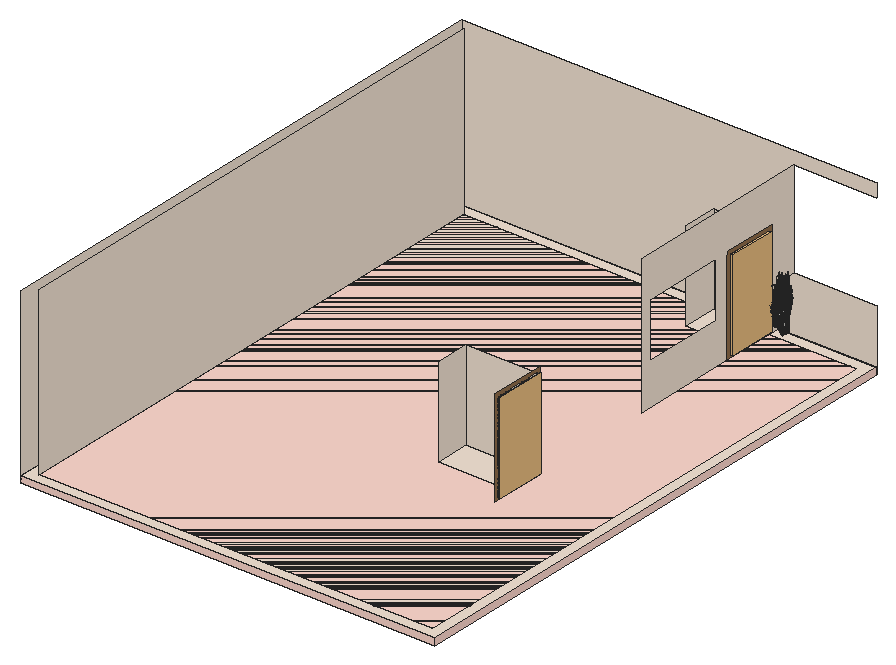
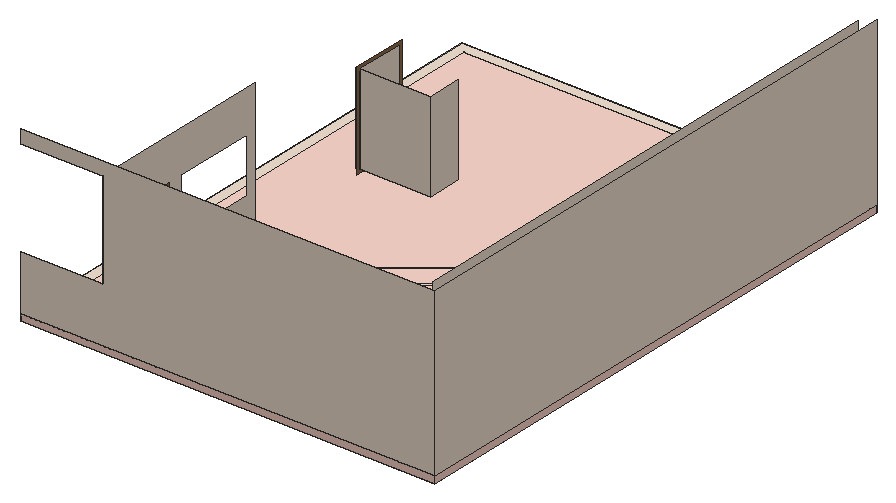
# SketchUp Ruby script. Lengths in inches.
U = 1.inch
M = Sketchup.active_model
def pt(a) = Geom::Point3d.new(a.map { |v| v * U })
def face(e, loops, mat)
  f = e.add_face(loops[0].map { |a| pt(a) })
  loops[1..].each { |l| e.add_face(l.map { |a| pt(a) }).erase! }
  f.material = f.back_material = mat if mat
  f
end
# faces: each face lists its corners as indices into pts; further lists are holes
def faces(e, pts, list, mat = nil) = list.each { |f| face(e, (f[0].is_a?(Array) ? f : [f]).map { |l| l.map { |i| pts[i] } }, mat) }
# xy, xz, yz: faces in a plane at the given z, y or x. An outline is a flat list of corners, or four numbers for a rectangle; further outlines are holes
def ring(l) = l.size == 4 ? [[l[0], l[1]], [l[2], l[1]], [l[2], l[3]], [l[0], l[3]]] : l.each_slice(2).to_a
def flat(e, list, mat, &to3) = list.each { |f| face(e, (f[0].is_a?(Array) ? f : [f]).map { |l| ring(l).map { |u, v| to3.(u, v) } }, mat) }
def xy(e, z, list, mat = nil) = flat(e, list, mat) { |x, y| [x, y, z] }
def xz(e, y, list, mat = nil) = flat(e, list, mat) { |x, z| [x, y, z] }
def yz(e, x, list, mat = nil) = flat(e, list, mat) { |y, z| [x, y, z] }
def lines(e, pts, list) = list.each { |a, b| e.add_line(pt(pts[a]), pt(pts[b])) }
# prism: a flat outline (further loops are holes) pulled along v
def prism(e, loops, v, mat = nil)
  f = face(e, loops, mat); d = Geom::Vector3d.new(v.map { |x| x * U })
  f.pushpull(f.normal.samedirection?(d) ? d.length : -d.length)
end
def box(e, o, s, mat = nil) = prism(e, [[o, [o[0] + s[0], o[1], o[2]], [o[0] + s[0], o[1] + s[1], o[2]], [o[0], o[1] + s[1], o[2]]]], [0, 0, s[2]], mat)
def at(x, y, z, deg = 0) = Geom::Transformation.translation(pt([x, y, z])) * Geom::Transformation.rotation(ORIGIN, Z_AXIS, deg.degrees)
def axes(o, x, y, z) = Geom::Transformation.new([*x, 0, *y, 0, *z, 0, *pt(o).to_a, 1])
def part(name) = M.definitions.add(name)
# library, detail: a bought-in or finely detailed component or shape, given as its bounding box
def library(name, o, s) = part(name).tap { |d| box(d.entities, o, s) }
def detail(e, o, s) = box(e.add_group.entities, o, s)
def put(e, d, t, mat = nil) = e.add_instance(d, t).tap { |i| i.material = mat if mat }
def group(e, t, mat = nil) = e.add_group.tap { |g| g.transformation = t; g.material = mat if mat }.entities
root = M.entities
M.materials.add("B01_Ivory_Dust").color = [255, 217, 206]
M.materials.add("C01_Vanilla_Cream").color = [244, 228, 212]
M.materials.add("LightPink_Translucent").color = [144, 107, 117]
M.materials["LightPink_Translucent"].alpha = 0.75
M.materials.add("Wood_Floor_01_1K").color = [146, 111, 76]
c1 = part("Group\#10")
box(c1.entities,[0,0,0],[360,480,6])
c2 = library("porta+4",[0.2,-5.42,1.33],[46.55,4.72,83.21])
c3 = part("blade")
p = [[2.15,0.21,22],[0,0.17,0],[0.09,0.45,0],[2.18,0.31,22],[2.29,0.31,22],[0.38,0.45,0],
  [2.48,0.24,33],[2.49,0.24,33],[2.48,0.22,33]]
faces(c3.entities,p,[[0,1,2,3],[4,5,2,3],[6,3,4,7],[8,0,3,6]])
c4 = part("seeds")
p = [[0.3,-0.1,1.38],[-0.01,-0.03,1.59],[-0.01,-0.03,0.03],[0.14,-0.07,-0.07],[0.29,-0.03,3],[0.15,0.01,3.11]]
faces(c4.entities,p,[[0,1,2,3],[1,0,4,5]],"LightPink_Translucent")
c5 = part("blade with seeds")
put(c5.entities,c3,at(0,0,0))
put(c5.entities,c4,axes([2.4,0.25,30.99],[1.5799,-0.05474,1.17369],[-0.12525,1.92788,0.29478],[-0.07173,-0.02425,1.56792]))
xy(root,96,[[288,324,290,396]],"C01_Vanilla_Cream")
xy(root,144,[[[0,0,360,480],[9,9,351,471]]],"C01_Vanilla_Cream")
xy(root,150,[[[0,0,360,480],[9,9,351,471]],[9,9,351,471]],"C01_Vanilla_Cream")
xy(root,165,[[226.53,171,288,201],[240,423,288,453]],"C01_Vanilla_Cream")
xz(root,201,[[226.53,165,288,243]],"C01_Vanilla_Cream")
xz(root,453,[[240,165,288,243]],"C01_Vanilla_Cream")
xz(root,480,[[0,150,0,294,360,294,360,282,288,282,288,198,360,198,360,150]],"C01_Vanilla_Cream")
yz(root,0,[[0,150,480,294]],"C01_Vanilla_Cream")
yz(root,9,[[9,150,471,294]],"C01_Vanilla_Cream")
yz(root,226.53,[[171,165,201,243]],"C01_Vanilla_Cream")
yz(root,240,[[423,165,453,243]],"C01_Vanilla_Cream")
yz(root,288,[[[314.71,162,408,162,408,246,456,246,456,162,468,162,468,198,480,198,480,282,314.71,282],[324,198,396,246]],[159,165,201,243],[411,165,453,243]],"C01_Vanilla_Cream")
yz(root,288,[[[156,162,204,246],[159,165,201,243]],[[408,162,456,246],[411,165,453,243]]],"Wood_Floor_01_1K")
put(root,c1,at(0,0,144),"B01_Ivory_Dust")
put(root,c2,axes([291.16,410.82,163.74],[0,0.8978,0],[0.58403,0,0],[0,0,0.94]),"C01_Vanilla_Cream")
put(root,c5,axes([295.36,458.6,164.91],[0.23093,-0.01116,1.28532],[-0.15319,0.4836,0.10393],[-0.32909,-0.02991,0.54946]))
put(root,c5,axes([295.45,459.45,164.91],[0.19317,-0.10421,1.28532],[0.16263,0.48153,0.10393],[-0.30326,0.10883,0.54946]))
put(root,c5,axes([294.85,460.27,163.94],[0.19348,0.04044,1.07251],[0.1247,0.41309,-0.23066],[-0.26282,0.07733,0.45856]))
put(root,c2,axes([289.83,157.29,163.73],[0,0.9504,0],[-0.24166,0,0],[0,0,0.9416]),"C01_Vanilla_Cream")
put(root,c5,axes([296.5625,458.95,164.51],[0.15825,-0.07127,1.32798],[0.05457,0.4976,0.10393],[-0.34278,0.06603,0.47463]))
put(root,c5,axes([294.86,459.28,165.54],[-0.09091,0.06396,1.31208],[0.00773,0.46734,-0.2075],[-0.20839,0.06078,0.10523]))
put(root,c5,axes([296.05,458.15,165.74],[-0.55654,-0.01186,-0.53284],[0.03738,-0.49951,0.0643],[-0.23578,-0.05271,0.75375]))
put(root,c5,axes([295.6,458.27,163.94],[0.1087,0.13716,1.07251],[-0.25048,0.37284,-0.23066],[-0.25719,-0.08912,0.45856]))
put(root,c5,axes([295.15,459.02,165.39],[-0.46269,-0.13744,-0.2656],[0.13495,-0.40096,0.3429],[-0.18628,0.03677,0.65611]))
put(root,c5,axes([295.79,457.83,164.91],[0.2068,0.08488,1.28532],[-0.42797,0.35609,0.10393],[-0.26673,-0.16064,0.54946]))
put(root,c5,axes([293.85,459.76,165.53],[0.07105,0.01321,1.33037],[0.2198,0.43529,-0.12571],[-0.14545,0.11425,0.23543]))
put(root,c5,axes([295.47,459.22,165.51],[-0.15083,0.44814,-0.38324],[-0.51712,-0.15361,-0.29685],[-0.2082,0.04109,0.7333]))
put(root,c5,axes([295.86,458.25,165.51],[-0.40426,0.32635,-0.38324],[-0.35404,-0.34474,-0.29685],[-0.2054,-0.04965,0.7333]))
put(root,c5,axes([295.21,459.19,163.12],[0.01412,0.07764,1.32257],[-0.28464,0.40547,-0.20205],[-0.20218,-0.02044,0.22528]))
put(root,c5,axes([295.29,457.34,165.53],[0.04127,0.04917,1.33037],[-0.19898,0.44196,-0.12571],[-0.20151,0.0032,0.23543]))
put(root,c5,axes([294.45,461.14,164.07],[0.23202,-0.22328,0.86145],[0.09155,0.35348,0.63294],[-0.16768,0.06329,0.18974]))
put(root,c5,axes([295.75,457.04,165.54],[-0.11979,-0.00348,1.31208],[-0.38137,0.34775,-0.2075],[-0.20349,-0.07106,0.10523]))
put(root,c5,axes([295.26,458.97,165.55],[0.15729,-0.44921,0.36002],[0.51712,0.15361,0.29685],[-0.20336,0.027,0.74497]))
put(root,c5,axes([295.44,458.84,165.78],[0.28012,0.44611,-0.0912],[-0.49717,0.21923,-0.50621],[-0.20951,0.05886,0.76918]))
put(root,c5,axes([296.07,457.91,165.78],[-0.02981,0.50103,-0.0912],[-0.56442,-0.01369,-0.50621],[-0.21738,-0.0348,0.76918]))
put(root,c5,axes([295.71,457.95,165.39],[-0.31678,-0.30846,-0.2656],[0.36171,-0.29199,0.3429],[-0.18378,-0.04443,0.65611]))
put(root,c5,axes([295.22,458.85,165.55],[-0.20448,-0.33592,0.04823],[0.37288,-0.16442,0.37966],[-0.16437,0.03244,0.57892]))
put(root,c5,axes([296.16,459.78,164.91],[0.13906,-0.15138,1.28532],[0.35111,0.40859,0.10393],[-0.24082,0.18608,0.54946]))
put(root,c5,axes([295.32,460.17,165.39],[-0.48462,0.07041,-0.2656],[-0.12797,-0.4025,0.3429],[-0.13888,0.10811,0.65611]))
put(root,c5,axes([295.06,461.37,163.12],[0.07468,0.04922,1.32257],[0.12663,0.45605,-0.20205],[-0.16551,0.09725,0.22528]))
put(root,c5,axes([294.95,458.6875,164.07],[0.35544,-0.03525,0.86145],[-0.22547,0.31061,0.63294],[-0.17565,-0.04659,0.18974]))
put(root,c5,axes([295.38,460.09,165.55],[-0.13808,-0.45342,0.36002],[0.54163,-0.07869,0.29685],[-0.15963,0.10664,0.74497]))
put(root,c5,axes([295.66,457.83,165.82],[0.45978,-0.36358,0.40322],[0.39653,0.38611,0.33247],[-0.21571,-0.06707,0.83437]))
put(root,c5,axes([295.28,460,165.55],[-0.3822,-0.20719,0.04823],[0.22252,-0.29505,0.37966],[-0.12254,0.09539,0.57892]))
put(root,c5,axes([296.05,460.15,164.91],[0.10366,-0.16934,1.28532],[0.43488,0.35044,0.10393],[-0.19618,0.21841,0.54946]))
put(root,c5,axes([295.64,458.97,165.79],[0.46269,0.13744,0.2656],[-0.13495,0.40096,-0.3429],[-0.18628,0.03677,0.65611]))
put(root,c5,axes([295.72,460.22,165.51],[0.14302,0.44985,-0.38324],[-0.54163,0.07869,-0.29685],[-0.15522,0.12083,0.7333]))
put(root,c5,axes([295.875,457.83,165.55],[0.02803,-0.37463,0.04823],[0.42332,0.01027,0.37966],[-0.16216,-0.0392,0.57892]))
put(root,c5,axes([294.875,461.03,165.54],[-0.01384,0.09749,1.31208],[0.39274,0.33916,-0.2075],[-0.10282,0.16039,0.10523]))
put(root,c5,axes([297.07,459.9,163.54],[-0.57914,-0.08077,-0.46765],[0.12221,-0.49823,-0.12274],[-0.17283,-0.06037,1.03225]))
put(root,c5,axes([297.18,457.18,166.07],[-0.37157,0.4723,-0.10215],[-0.5381,-0.2721,-0.56695],[-0.18705,-0.13344,0.86148]))
put(root,c5,axes([296.16,458.11,165.79],[0.31678,0.30846,0.2656],[-0.36171,0.29199,-0.3429],[-0.18378,-0.04443,0.65611]))
put(root,c5,axes([297.01,457.5625,165.74],[-0.47473,-0.23813,-0.53284],[0.33738,-0.41728,0.0643],[-0.172,-0.14218,0.75375]))
put(root,c5,axes([296.79,457.58,165.51],[-0.54938,0.11711,-0.38324],[-0.0961,-0.44351,-0.29685],[-0.14756,-0.1271,0.7333]))
put(root,c5,axes([296.3125,460.84,163.51],[-0.52105,-0.24633,-0.37238],[0.31144,-0.44171,0],[-0.11867,-0.0561,1.18128]))
put(root,c5,axes([296.08,457.17,163.12],[-0.05393,0.0649,1.32257],[-0.545,0.13993,-0.20205],[-0.13166,-0.12729,0.22528]))
put(root,c5,axes([295.47,459.9,165.78],[0.515,0.27165,-0.0912],[-0.2967,0.3934,-0.50621],[-0.1455,0.13675,0.76918]))
put(root,c5,axes([296.63,461.14,163.78],[-0.34808,0.49367,0],[-0.58235,-0.27531,-0.38706],[-0.13264,-0.0627,1.22783]))
put(root,c5,axes([294.62,461.08,166.23],[0.49129,0.13151,-0.04866],[-0.15113,0.40475,-0.22062],[-0.08035,0.06145,0.72768]))
put(root,c5,axes([295.72,459.94,165.79],[0.48462,-0.07041,0.2656],[0.12797,0.4025,-0.3429],[-0.13888,0.10811,0.65611]))
put(root,c5,axes([295.99,461.85,163.94],[0.17569,-0.07772,1.07251],[0.43377,0.23434,-0.23066],[-0.12911,0.20277,0.45856]))
put(root,c5,axes([295.74,457.42,163.6],[-0.1606,0.40228,-0.02919],[-0.4943,-0.12375,-0.13237],[-0.07505,-0.0658,0.43661]))
put(root,c5,axes([297.03,456.06,165.53],[-0.01039,0.05905,1.33037],[-0.51226,0.21431,-0.12571],[-0.15074,-0.10955,0.23543]))
put(root,c5,axes([296.48,456.91,163.94],[-0.03371,0.16116,1.07251],[-0.49286,0.13491,-0.23066],[-0.11521,-0.20831,0.45856]))
put(root,c5,axes([296.64,457.33,164.91],[0.12726,0.15818,1.28532],[-0.58807,0.13317,0.10393],[-0.13291,-0.24832,0.54946]))
put(root,c5,axes([297.73,459.97,164],[-0.56211,0.32708,-0.21822],[-0.3738,-0.46216,-0.37502],[-0.13869,-0.04694,1.19781]))
put(root,c5,axes([296.18,461,165.55],[-0.39645,-0.33614,0.36002],[0.42102,-0.2899,0.29685],[-0.07313,0.15771,0.74497]))
put(root,c5,axes([296.85,457.25,165.39],[-0.08599,-0.39682,-0.2656],[0.49155,-0.10478,0.3429],[-0.13203,-0.11372,0.65611]))
put(root,c5,axes([295.48,459.26,163.78],[-0.69617,0,0],[0,-0.55062,-0.38706],[0,-0.12541,1.22783]))
put(root,c5,axes([296.46,460.66,163.52],[-0.13078,-0.42928,-0.23233],[0.51941,-0.1219,0.23233],[-0.10471,-0.0495,1.0423]))
put(root,c5,axes([296.03,460.97,165.55],[-0.45752,-0.02296,0.04823],[0.01254,-0.34663,0.37966],[-0.04787,0.13278,0.57892]))
put(root,c5,axes([296.17,461.1,165.39],[-0.3767,0.25939,-0.2656],[-0.3566,-0.29618,0.3429],[-0.05426,0.15048,0.65611]))
put(root,c5,axes([298.1,460.33,163.54],[-0.375,0.3703,-0.46765],[-0.46584,-0.33578,-0.12274],[-0.15027,0.09237,1.03225]))
put(root,c5,axes([297.14,457.57,165.79],[0.08599,0.39682,0.2656],[-0.49155,0.10478,-0.3429],[-0.13203,-0.11372,0.65611]))
put(root,c5,axes([294.83,462.03,165.53],[0.06316,-0.02974,1.33037],[0.52204,0.19785,-0.12571],[-0.01227,0.16473,0.23543]))
put(root,c5,axes([296.02,459.11,163.75],[-0.51786,0.4142,0.23067],[-0.51817,-0.40984,-0.27369],[-0.01808,-0.11762,1.23664]))
put(root,c5,axes([298.15,460.26,164.49],[0.48111,0.19866,1.13446],[-0.47133,0.42798,0.44862],[-0.21112,-0.25366,0.95105]))
put(root,c5,axes([296.3125,456.65,164.07],[0.29042,0.17147,0.86145],[-0.42295,0.10307,0.63294],[-0.0905,-0.13178,0.18974]))
put(root,c5,axes([298.36,460.12,163.85],[-0.54364,-0.39653,-0.18894],[0.45745,-0.44527,0.41347],[-0.14639,0.04639,1.26162]))
put(root,c5,axes([297.37,459.74,163.66],[-0.33445,-0.41351,-0.33554],[0.50659,-0.29119,0.16149],[-0.10823,-0.05117,1.07733]))
put(root,c5,axes([296.43,460.83,166],[-0.01449,0.45571,-0.59145],[-0.61002,-0.03061,0.07138],[-0.06438,0.19306,0.83667]))
put(root,c5,axes([296.41,462.11,164.07],[-0.01441,-0.29294,0.86145],[0.36003,0.20894,0.63294],[-0.07081,0.13963,0.18974]))
put(root,c5,axes([296.92,457.1,165.82],[0.62019,-0.12663,0.40322],[0.10763,0.49673,0.33247],[-0.14586,-0.1464,0.83437]))
put(root,c5,axes([298.08,460.04,163.66],[-0.60457,0.03041,-0.33554],[-0.05467,-0.50484,0.16149],[-0.10823,0.05117,1.07733]))
put(root,c5,axes([297.0625,457.21,165.55],[0.25304,-0.31296,0.04823],[0.36033,0.18221,0.37966],[-0.11649,-0.10034,0.57892]))
put(root,c5,axes([296.93,460.88,163.86],[0.52105,0.24633,0.37238],[-0.31144,0.44171,0],[-0.11867,-0.0561,1.18128]))
put(root,c5,axes([296.22,461.47,164.52],[0.01223,-0.25433,1.15759],[0.55017,0.13434,0.15997],[-0.04767,0.27105,0.54661]))
put(root,c5,axes([297.42,459.98,163.83],[0.14756,-0.58378,-0.17572],[0.69966,0.10176,0.38453],[-0.12225,-0.08062,1.1733]))
put(root,c5,axes([297.68,460.11,163.96],[-0.1074,0.43968,0.1086],[-0.52474,-0.07632,-0.3101],[-0.0955,-0.04515,0.95058]))
put(root,c5,axes([297.61,456.28,165.54],[-0.08515,-0.06907,1.31208],[-0.56828,0.04379,-0.2075],[-0.0907,-0.16522,0.10523]))
put(root,c5,axes([298.72,461.34,163.51],[-0.52105,0.24633,-0.37238],[-0.31144,-0.44171,0],[-0.11867,0.0561,1.18128]))
put(root,c5,axes([295.63,458.88,163.51],[0,-0.49266,-0.37238],[0.62289,0,0],[0,-0.11221,1.18128]))
put(root,c5,axes([295.9,459.34,163.86],[0,0.49266,0.37238],[-0.62289,0,0],[0,-0.11221,1.18128]))
put(root,c5,axes([298.75,461.21,163.64],[-0.34375,-0.4954,-0.03857],[0.58235,-0.27531,0.38706],[-0.1435,0.04717,1.22723]))
put(root,c5,axes([296.55,460.98,165.75],[0.39855,0.33102,-0.4254],[-0.42102,0.2899,-0.32951],[-0.06064,0.16819,0.81396]))
put(root,c5,axes([298.6,461.14,163.52],[-0.51941,-0.1219,-0.23233],[0.13078,-0.42928,0.23233],[-0.10471,0.0495,1.0423]))
put(root,c5,axes([296.37,460.74,165.79],[0.3767,-0.25939,0.2656],[0.3566,0.29618,-0.3429],[-0.05426,0.15048,0.65611]))
put(root,c5,axes([297.26,459.45,164],[-0.62699,-0.23507,-0.21822],[0.3019,-0.49615,-0.37502],[-0.0197,-0.12182,1.19781]))
put(root,c5,axes([298.9,459.31,164.13],[-0.01521,-0.46386,1.05954],[0.68831,0.12024,0.44862],[-0.1628,0.25382,1.00012]))
put(root,c5,axes([296.13,460.81,166.05],[0.61188,0.02441,-0.10123],[-0.01672,0.46217,-0.56189],[-0.0425,0.178,0.85379]))
put(root,c5,axes([296.12,461.48,164.12],[0.50577,-0.08724,0.04881],[0.11627,0.35148,-0.64728],[-0.03206,0.17792,0.5802]))
put(root,c5,axes([298.51,459.9,164],[0.06488,0.56215,-0.21822],[-0.6757,0.03399,-0.37502],[-0.11898,0.07488,1.19781]))
put(root,c5,axes([296.98,458.95,163.57],[-0.22864,-0.5052,-0.52377],[0.65862,-0.18195,-0.13747],[-0.02527,-0.17107,1.15612]))
put(root,c5,axes([298.48,457.35,165.78],[-0.54481,0.22937,-0.0912],[-0.26773,-0.4071,-0.50621],[-0.07188,-0.17155,0.76918]))
put(root,c5,axes([298.01,457.37,165.51],[-0.54728,-0.1235,-0.38324],[0.18759,-0.42344,-0.29685],[-0.05018,-0.17048,0.7333]))
put(root,c5,axes([297,460.51,164.91],[-0.01363,-0.18909,1.28532],[0.5906,0.12544,0.10393],[-0.03653,0.26947,0.54946]))
put(root,c5,axes([295.9,458.89,163.52],[0.38863,-0.30738,-0.23233],[0.38863,0.30738,0.23233],[0,-0.09901,1.0423]))
put(root,c5,axes([297.66,456.91,163.6],[-0.38473,0.28263,-0.02919],[-0.35252,-0.30954,-0.13237],[-0.02482,-0.08771,0.43661]))
put(root,c5,axes([297.5,459.69,163.77],[0.70367,0.1038,0.34316],[-0.1432,0.58624,0.13466],[-0.10283,-0.05661,1.19142]))
put(root,c5,axes([297.32,459.59,164.04],[-0.27012,0.44393,0.33554],[-0.56127,-0.21365,-0.16149],[0,-0.10233,1.07733]))
put(root,c5,axes([298.21,457.45,165.74],[-0.26572,-0.40059,-0.53284],[0.54698,-0.22325,0.0643],[-0.06214,-0.19355,0.75375]))
put(root,c5,axes([297.125,460.63,163.86],[0.59825,-0.13076,0.13232],[0.14773,0.48663,0.26315],[-0.05336,-0.0709,1.20305]))
put(root,c5,axes([297.89,460.71,163.65],[-0.56127,-0.22118,0],[0.27012,-0.45959,0],[0,0,1.2203]))
put(root,c5,axes([298.32,457.51,165.79],[-0.16784,0.37886,0.2656],[-0.48968,-0.1105,-0.3429],[-0.0449,-0.15254,0.65611]))
put(root,c5,axes([299.19,461.26,163.78],[0.34808,0.49367,0],[-0.58235,0.27531,-0.38706],[-0.13264,0.0627,1.22783]))
put(root,c5,axes([297.42,461.47,165.8],[-0.54859,-0.1288,0.39962],[0.18759,-0.42344,0.32951],[0.03297,0.16652,0.82692]))
put(root,c5,axes([297.28,461.51,165.55],[-0.41024,0.16744,0.04823],[-0.2008,-0.30532,0.37966],[0.03962,0.13459,0.57892]))
put(root,c5,axes([298.9,460.66,163.86],[0.16083,-0.48962,0.13232],[0.58854,0.13856,0.26315],[-0.10167,0.00238,1.20305]))
put(root,c5,axes([298.63,460.01,163.96],[0.41131,0.296,0.1086],[-0.34309,0.33395,-0.3101],[-0.0955,0.04515,0.95058]))
put(root,c5,axes([298.49,459.64,163.72],[-0.51786,-0.42404,-0.04598],[0.51817,-0.4243,0],[-0.01808,-0.01481,1.31678]))
put(root,c5,axes([298.62,459.79,164.04],[0.60457,-0.03041,0.33554],[0.05467,0.50484,-0.16149],[-0.10823,0.05117,1.07733]))
put(root,c5,axes([298.77,460.95,163.75],[0.697,0.16013,0.23067],[-0.17437,0.57237,-0.27369],[-0.11536,0.07164,1.23664]))
put(root,c5,axes([297.75,456.5625,163.12],[-0.09338,0.01775,1.32257],[-0.51641,-0.1998,-0.20205],[0.00867,-0.16666,0.22528]))
put(root,c5,axes([299.07,460.92,163.86],[0.52105,-0.24633,0.37238],[0.31144,0.44171,0],[-0.11867,0.0561,1.18128]))
put(root,c5,axes([298.26,457.11,165.39],[0.16784,-0.37886,-0.2656],[0.48968,0.1105,0.3429],[-0.0449,-0.15254,0.65611]))
put(root,c5,axes([297.44,459.16,163.77],[0.24206,0.5509,0.34316],[-0.69162,0.19157,0.13466],[0.00845,-0.10123,1.19142]))
put(root,c5,axes([297.33,459.09,163.66],[0.27012,-0.44393,-0.33554],[0.56127,0.21365,0.16149],[0,-0.10233,1.07733]))
put(root,c5,axes([298.02,460.52,163.65],[-0.18165,-0.42474,0],[0.51872,-0.14874,0],[0,0,1.15778]))
